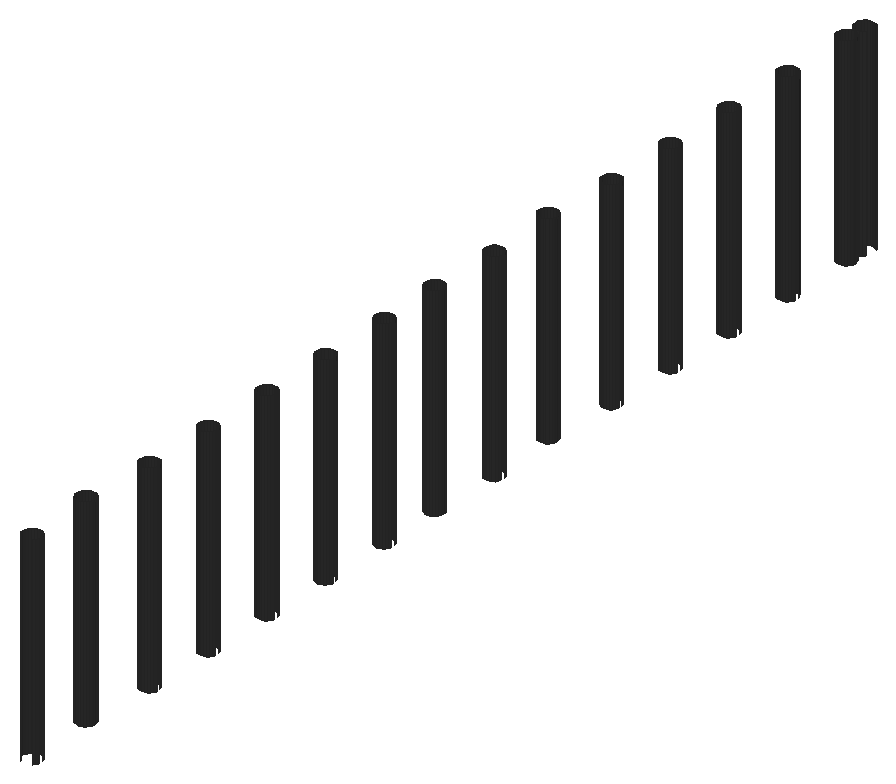
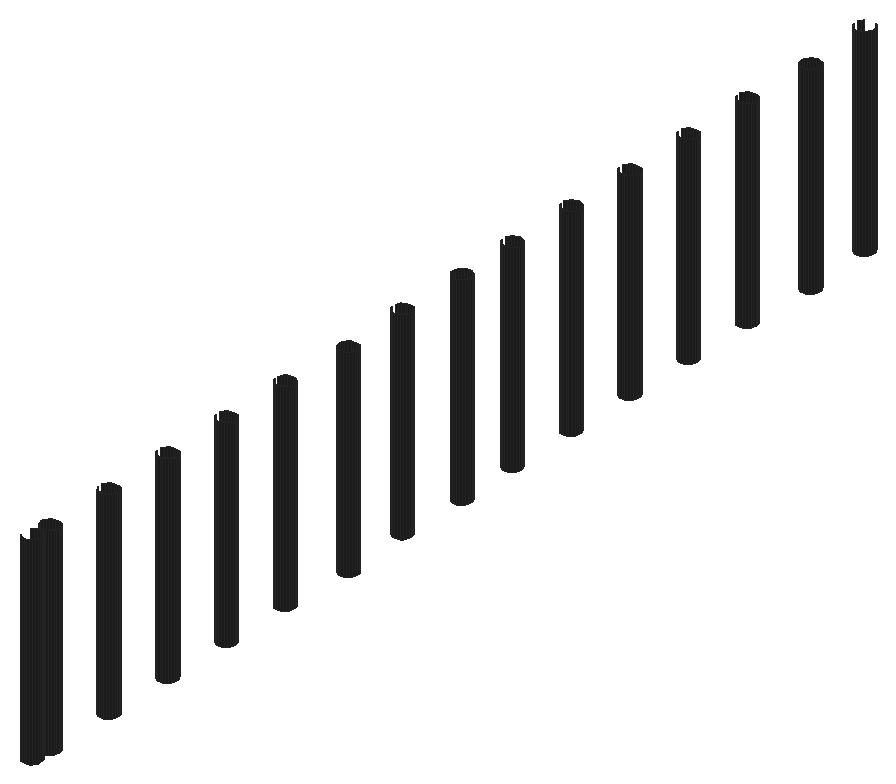
# SketchUp Ruby script. Lengths in inches.
U = 1.inch
M = Sketchup.active_model
def pt(a) = Geom::Point3d.new(a.map { |v| v * U })
def face(e, loops, mat)
  f = e.add_face(loops[0].map { |a| pt(a) })
  loops[1..].each { |l| e.add_face(l.map { |a| pt(a) }).erase! }
  f.material = f.back_material = mat if mat
  f
end
# faces: each face lists its corners as indices into pts; further lists are holes
def faces(e, pts, list, mat = nil) = list.each { |f| face(e, (f[0].is_a?(Array) ? f : [f]).map { |l| l.map { |i| pts[i] } }, mat) }
# xy, xz, yz: faces in a plane at the given z, y or x. An outline is a flat list of corners, or four numbers for a rectangle; further outlines are holes
def ring(l) = l.size == 4 ? [[l[0], l[1]], [l[2], l[1]], [l[2], l[3]], [l[0], l[3]]] : l.each_slice(2).to_a
def flat(e, list, mat, &to3) = list.each { |f| face(e, (f[0].is_a?(Array) ? f : [f]).map { |l| ring(l).map { |u, v| to3.(u, v) } }, mat) }
def xy(e, z, list, mat = nil) = flat(e, list, mat) { |x, y| [x, y, z] }
def xz(e, y, list, mat = nil) = flat(e, list, mat) { |x, z| [x, y, z] }
def yz(e, x, list, mat = nil) = flat(e, list, mat) { |y, z| [x, y, z] }
def lines(e, pts, list) = list.each { |a, b| e.add_line(pt(pts[a]), pt(pts[b])) }
# prism: a flat outline (further loops are holes) pulled along v
def prism(e, loops, v, mat = nil)
  f = face(e, loops, mat); d = Geom::Vector3d.new(v.map { |x| x * U })
  f.pushpull(f.normal.samedirection?(d) ? d.length : -d.length)
end
def box(e, o, s, mat = nil) = prism(e, [[o, [o[0] + s[0], o[1], o[2]], [o[0] + s[0], o[1] + s[1], o[2]], [o[0], o[1] + s[1], o[2]]]], [0, 0, s[2]], mat)
def at(x, y, z, deg = 0) = Geom::Transformation.translation(pt([x, y, z])) * Geom::Transformation.rotation(ORIGIN, Z_AXIS, deg.degrees)
def axes(o, x, y, z) = Geom::Transformation.new([*x, 0, *y, 0, *z, 0, *pt(o).to_a, 1])
def part(name) = M.definitions.add(name)
# library, detail: a bought-in or finely detailed component or shape, given as its bounding box
def library(name, o, s) = part(name).tap { |d| box(d.entities, o, s) }
def detail(e, o, s) = box(e.add_group.entities, o, s)
def put(e, d, t, mat = nil) = e.add_instance(d, t).tap { |i| i.material = mat if mat }
def group(e, t, mat = nil) = e.add_group.tap { |g| g.transformation = t; g.material = mat if mat }.entities
root = M.entities
M.materials.add("[0137_Black]").color = [45, 45, 45]
p = [[2.88,315.04,48],[3.5,314.56,48],[3.5,314.56,113.8],[2.88,315.04,113.8],[2.4,315.66,48],[2.4,315.66,113.8],
  [7.125,315.04,48],[7.6,315.66,48],[7.6,315.66,113.8],[7.125,315.04,113.8],[2.11,316.38,48],[2.11,316.38,113.8],
  [7.9,316.38,48],[7.9,316.38,113.8],[2,317.16,48],[2,317.16,113.8],[2.11,317.93,48],[2.11,317.93,113.8],
  [2.4,318.66,48],[2.4,318.66,113.8],[7.9,317.93,48],[7.6,318.66,48],[7.6,318.66,113.8],[7.9,317.93,113.8],
  [2.88,319.28,48],[2.88,319.28,113.8],[7.125,319.28,48],[7.125,319.28,113.8],[3.5,319.76,48],[3.5,319.76,113.8],
  [6.5,319.76,48],[6.5,319.76,113.8],[4.23,320.06,48],[4.23,320.06,113.8],[4.23,320.06,113.61],[5.78,320.06,48],
  [5.78,320.06,113.8],[5,320.16,48],[5,320.16,113.8],[5,320.16,113.71],[2.67,338.26,48],[3.45,338.16,48],
  [3.45,338.16,113.71],[3.45,338.16,113.8],[2.67,338.26,113.8],[4.23,338.26,48],[4.23,338.26,113.61],[4.23,338.26,113.8],
  [1.95,338.56,48],[1.95,338.56,113.8],[4.95,338.56,48],[4.95,338.56,113.8],[1.33,339.04,48],[1.33,339.04,113.8],
  [5,338.6,48],[5.57,339.04,48],[5.57,339.04,113.8],[0.85,339.66,48],[0.85,339.66,113.8],[6.05,339.66,48],
  [6.05,339.66,113.8],[0.55,340.38,48],[0.55,340.38,113.8],[6.35,340.38,48],[6.35,340.38,113.8],[0.45,341.16,48],
  [0.45,341.16,113.8],[6.45,341.16,48],[6.45,341.16,113.8],[0.55,341.93,48],[0.55,341.93,113.8],[6.35,341.93,48],
  [6.35,341.93,113.8],[0.85,342.66,48],[0.85,342.66,113.8],[6.05,342.66,48],[6.05,342.66,113.8],[1.33,343.28,48],
  [1.33,343.28,113.8],[5.57,343.28,48],[5.57,343.28,113.8],[1.95,343.76,48],[1.95,343.76,113.8],[5,343.72,48],
  [4.95,343.76,48],[4.95,343.76,113.8],[2.67,344.06,48],[2.67,344.06,113.8],[4.23,344.06,48],[4.23,344.06,113.61],
  [4.23,344.06,113.8],[3.45,344.16,48],[3.45,344.16,113.8],[3.45,344.16,113.71],[4.23,362.26,48],[5,362.16,48],
  [5,362.16,113.71],[5,362.16,113.8],[4.23,362.26,113.8],[4.23,362.26,113.61],[5.78,362.26,48],[5.78,362.26,113.8],
  [3.5,362.56,48],[3.5,362.56,113.8],[6.5,362.56,48],[6.5,362.56,113.8],[2.88,363.04,48],[2.88,363.04,113.8],
  [7.125,363.04,48],[7.125,363.04,113.8],[2.4,363.66,48],[2.4,363.66,113.8],[7.6,363.66,48],[7.6,363.66,113.8],
  [2.11,364.38,48],[2.11,364.38,113.8],[7.9,364.38,48],[7.9,364.38,113.8],[2,365.16,48],[2,365.16,113.8],
  [2.11,365.93,48],[2.11,365.93,113.8],[2.4,366.66,48],[2.4,366.66,113.8],[7.9,365.93,48],[7.6,366.66,48],
  [7.6,366.66,113.8],[7.9,365.93,113.8],[2.88,367.28,48],[2.88,367.28,113.8],[7.125,367.28,48],[7.125,367.28,113.8],
  [3.5,367.76,48],[3.5,367.76,113.8],[6.5,367.76,48],[6.5,367.76,113.8],[4.23,368.06,48],[4.23,368.06,113.8],
  [4.23,368.06,113.61],[5.78,368.06,48],[5.78,368.06,113.8],[5,368.16,48],[5,368.16,113.8],[5,368.16,113.71],
  [4.23,386.26,48],[5,386.16,48],[5,386.16,113.71],[5,386.16,113.8],[4.23,386.26,113.8],[4.23,386.26,113.61],
  [5.78,386.26,48],[5.78,386.26,113.8],[3.5,386.56,48],[3.5,386.56,113.8],[6.5,386.56,48],[6.5,386.56,113.8],
  [2.88,387.04,48],[2.88,387.04,113.8],[7.125,387.04,48],[7.125,387.04,113.8],[2.4,387.66,48],[2.4,387.66,113.8],
  [7.6,387.66,48],[7.6,387.66,113.8],[2.11,388.38,48],[2.11,388.38,113.8],[7.9,388.38,48],[7.9,388.38,113.8],
  [2,389.16,48],[2,389.16,113.8],[2.11,389.93,48],[2.11,389.93,113.8],[2.4,390.66,48],[2.4,390.66,113.8],
  [7.9,389.93,48],[7.6,390.66,48],[7.6,390.66,113.8],[7.9,389.93,113.8],[2.88,391.28,48],[2.88,391.28,113.8],
  [7.125,391.28,48],[7.125,391.28,113.8],[3.5,391.76,48],[3.5,391.76,113.8],[6.5,391.76,48],[6.5,391.76,113.8],
  [4.23,392.06,48],[4.23,392.06,113.8],[4.23,392.06,113.61],[5.78,392.06,48],[5.78,392.06,113.8],[5,392.16,48],
  [5,392.16,113.8],[5,392.16,113.71],[4.23,410.26,48],[5,410.16,48],[5,410.16,113.71],[5,410.16,113.8],
  [4.23,410.26,113.8],[4.23,410.26,113.61],[5.78,410.26,48],[5.78,410.26,113.8],[3.5,410.56,48],[3.5,410.56,113.8],
  [6.5,410.56,48],[6.5,410.56,113.8],[2.88,411.04,48],[2.88,411.04,113.8],[7.125,411.04,48],[7.125,411.04,113.8],
  [2.4,411.66,48],[2.4,411.66,113.8],[7.6,411.66,48],[7.6,411.66,113.8],[2.11,412.38,48],[2.11,412.38,113.8],
  [7.9,412.38,48],[7.9,412.38,113.8],[2,413.16,48],[2,413.16,113.8],[2.11,413.93,48],[2.11,413.93,113.8],
  [2.4,414.66,48],[2.4,414.66,113.8],[7.9,413.93,48],[7.6,414.66,48],[7.6,414.66,113.8],[7.9,413.93,113.8],
  [2.88,415.28,48],[2.88,415.28,113.8],[7.125,415.28,48],[7.125,415.28,113.8],[3.5,415.76,48],[3.5,415.76,113.8],
  [6.5,415.76,48],[6.5,415.76,113.8],[4.23,416.06,48],[4.23,416.06,113.8],[4.23,416.06,113.61],[5.78,416.06,48],
  [5.78,416.06,113.8],[5,416.16,48],[5,416.16,113.8],[5,416.16,113.71],[4.23,434.26,48],[5,434.16,48],
  [5,434.16,113.71],[5,434.16,113.8],[4.23,434.26,113.8],[4.23,434.26,113.61],[5.78,434.26,48],[5.78,434.26,113.8],
  [3.5,434.56,48],[3.5,434.56,113.8],[6.5,434.56,48],[6.5,434.56,113.8],[2.88,435.04,48],[2.88,435.04,113.8],
  [7.125,435.04,48],[7.125,435.04,113.8],[2.4,435.66,48],[2.4,435.66,113.8],[7.6,435.66,48],[7.6,435.66,113.8],
  [2.11,436.38,48],[2.11,436.38,113.8],[7.9,436.38,48],[7.9,436.38,113.8],[2,437.16,48],[2,437.16,113.8],
  [2.11,437.93,48],[2.11,437.93,113.8],[2.4,438.66,48],[2.4,438.66,113.8],[7.9,437.93,48],[7.6,438.66,48],
  [7.6,438.66,113.8],[7.9,437.93,113.8],[2.88,439.28,48],[2.88,439.28,113.8],[7.125,439.28,48],[7.125,439.28,113.8],
  [3.5,439.76,48],[3.5,439.76,113.8],[6.5,439.76,48],[6.5,439.76,113.8],[4.23,440.06,48],[4.23,440.06,113.8],
  [4.23,440.06,113.61],[5.78,440.06,48],[5.78,440.06,113.8],[5,440.16,48],[5,440.16,113.8],[5,440.16,113.71],
  [4.23,458.26,48],[5,458.16,48],[5,458.16,113.71],[5,458.16,113.8],[4.23,458.26,113.8],[4.23,458.26,113.61],
  [5.78,458.26,48],[5.78,458.26,113.8],[3.5,458.56,48],[3.5,458.56,113.8],[6.5,458.56,48],[6.5,458.56,113.8],
  [2.88,459.04,48],[2.88,459.04,113.8],[7.125,459.04,48],[7.125,459.04,113.8],[2.4,459.66,48],[2.4,459.66,113.8],
  [7.6,459.66,48],[7.6,459.66,113.8],[2.11,460.38,48],[2.11,460.38,113.8],[7.9,460.38,48],[7.9,460.38,113.8],
  [2,461.16,48],[2,461.16,113.8],[2.11,461.93,48],[2.11,461.93,113.8],[2.4,462.66,48],[2.4,462.66,113.8],
  [7.9,461.93,48],[7.6,462.66,48],[7.6,462.66,113.8],[7.9,461.93,113.8],[2.88,463.28,48],[2.88,463.28,113.8],
  [7.125,463.28,48],[7.125,463.28,113.8],[3.5,463.76,48],[3.5,463.76,113.8],[6.5,463.76,48],[6.5,463.76,113.8],
  [4.23,464.06,48],[4.23,464.06,113.8],[4.23,464.06,113.61],[5.78,464.06,48],[5.78,464.06,113.8],[5,464.16,48],
  [5,464.16,113.8],[5,464.16,113.71],[3.61,479.625,48],[4.38,479.52,48],[4.38,479.52,113.8],[3.61,479.625,113.8],
  [5,479.61,48],[5.16,479.625,48],[5.16,479.625,113.8],[2.88,479.93,48],[2.88,479.93,113.8],[5.88,479.93,48],
  [5.88,479.93,113.8],[2.26,480.4,48],[2.26,480.4,113.8],[6.5,480.4,48],[6.5,480.4,113.8],[1.78,481.02,48],
  [1.78,481.02,113.8],[6.98,481.02,48],[6.98,481.02,113.8],[1.48,481.75,48],[1.48,481.75,113.8],[7.28,481.75,48],
  [7.28,481.75,113.8],[1.38,482.52,48],[1.38,482.52,113.8],[7.38,482.52,48],[7.38,482.52,113.8],[1.48,483.3,48],
  [1.48,483.3,113.8],[7.28,483.3,48],[7.28,483.3,113.8],[1.78,484.02,48],[1.78,484.02,113.8],[6.98,484.02,48],
  [6.98,484.02,113.8],[2.26,484.64,48],[2.26,484.64,113.8],[6.5,484.64,48],[6.5,484.64,113.8],[2.88,485.12,48],
  [2.88,485.12,113.8],[5.88,485.12,48],[5.88,485.12,113.8],[3.61,485.42,48],[3.61,485.42,113.8],[5.16,485.42,48],
  [5.16,485.42,113.8],[4.38,485.52,48],[4.38,485.52,113.8],[5,485.44,48],[4.23,503.15,48],[5,503.05,48],
  [5,503.05,113.71],[5,503.05,113.8],[4.23,503.15,113.8],[4.23,503.15,113.61],[5.78,503.15,48],[5.78,503.15,113.8],
  [3.5,503.45,48],[3.5,503.45,113.8],[6.5,503.45,48],[6.5,503.45,113.8],[2.88,503.93,48],[2.88,503.93,113.8],
  [7.125,503.93,48],[7.125,503.93,113.8],[2.4,504.55,48],[2.4,504.55,113.8],[7.6,504.55,48],[7.6,504.55,113.8],
  [2.11,505.27,48],[2.11,505.27,113.8],[7.9,505.27,48],[7.9,505.27,113.8],[2,506.05,48],[2,506.05,113.8],
  [2.11,506.82,48],[2.11,506.82,113.8],[2.4,507.55,48],[2.4,507.55,113.8],[7.9,506.82,48],[7.6,507.55,48],
  [7.6,507.55,113.8],[7.9,506.82,113.8],[2.88,508.17,48],[2.88,508.17,113.8],[7.125,508.17,48],[7.125,508.17,113.8],
  [3.5,508.64,48],[3.5,508.64,113.8],[6.5,508.64,48],[6.5,508.64,113.8],[4.23,508.94,48],[4.23,508.94,113.8],
  [4.23,508.94,113.61],[5.78,508.94,48],[5.78,508.94,113.8],[5,509.05,48],[5,509.05,113.8],[5,509.05,113.71],
  [2.67,527.15,48],[3.45,527.05,48],[3.45,527.05,113.71],[3.45,527.05,113.8],[2.67,527.15,113.8],[4.23,527.15,48],
  [4.23,527.15,113.61],[4.23,527.15,113.8],[1.95,527.45,48],[1.95,527.45,113.8],[4.95,527.45,48],[4.95,527.45,113.8],
  [1.33,527.93,48],[1.33,527.93,113.8],[5,527.49,48],[5.57,527.93,48],[5.57,527.93,113.8],[0.85,528.55,48],
  [0.85,528.55,113.8],[6.05,528.55,48],[6.05,528.55,113.8],[0.55,529.27,48],[0.55,529.27,113.8],[6.35,529.27,48],
  [6.35,529.27,113.8],[0.45,530.05,48],[0.45,530.05,113.8],[6.45,530.05,48],[6.45,530.05,113.8],[0.55,530.82,48],
  [0.55,530.82,113.8],[6.35,530.82,48],[6.35,530.82,113.8],[0.85,531.55,48],[0.85,531.55,113.8],[6.05,531.55,48],
  [6.05,531.55,113.8],[1.33,532.17,48],[1.33,532.17,113.8],[5.57,532.17,48],[5.57,532.17,113.8],[1.95,532.64,48],
  [1.95,532.64,113.8],[5,532.6,48],[4.95,532.64,48],[4.95,532.64,113.8],[2.67,532.94,48],[2.67,532.94,113.8],
  [4.23,532.94,48],[4.23,532.94,113.61],[4.23,532.94,113.8],[3.45,533.05,48],[3.45,533.05,113.8],[3.45,533.05,113.71],
  [4.23,551.15,48],[5,551.05,48],[5,551.05,113.71],[5,551.05,113.8],[4.23,551.15,113.8],[4.23,551.15,113.61],
  [5.78,551.15,48],[5.78,551.15,113.8],[3.5,551.45,48],[3.5,551.45,113.8],[6.5,551.45,48],[6.5,551.45,113.8],
  [2.88,551.93,48],[2.88,551.93,113.8],[7.125,551.93,48],[7.125,551.93,113.8],[2.4,552.55,48],[2.4,552.55,113.8],
  [7.6,552.55,48],[7.6,552.55,113.8],[2.11,553.27,48],[2.11,553.27,113.8],[7.9,553.27,48],[7.9,553.27,113.8],
  [2,554.05,48],[2,554.05,113.8],[2.11,554.82,48],[2.11,554.82,113.8],[2.4,555.55,48],[2.4,555.55,113.8],
  [7.9,554.82,48],[7.6,555.55,48],[7.6,555.55,113.8],[7.9,554.82,113.8],[2.88,556.17,48],[2.88,556.17,113.8],
  [7.125,556.17,48],[7.125,556.17,113.8],[3.5,556.64,48],[3.5,556.64,113.8],[6.5,556.64,48],[6.5,556.64,113.8],
  [4.23,556.94,48],[4.23,556.94,113.8],[4.23,556.94,113.61],[5.78,556.94,48],[5.78,556.94,113.8],[5,557.05,48],
  [5,557.05,113.8],[5,557.05,113.71],[4.23,575.15,48],[5,575.05,48],[5,575.05,113.71],[5,575.05,113.8],
  [4.23,575.15,113.8],[4.23,575.15,113.61],[5.78,575.15,48],[5.78,575.15,113.8],[3.5,575.45,48],[3.5,575.45,113.8],
  [6.5,575.45,48],[6.5,575.45,113.8],[2.88,575.93,48],[2.88,575.93,113.8],[7.125,575.93,48],[7.125,575.93,113.8],
  [2.4,576.55,48],[2.4,576.55,113.8],[7.6,576.55,48],[7.6,576.55,113.8],[2.11,577.27,48],[2.11,577.27,113.8],
  [7.9,577.27,48],[7.9,577.27,113.8],[2,578.05,48],[2,578.05,113.8],[2.11,578.82,48],[2.11,578.82,113.8],
  [2.4,579.55,48],[2.4,579.55,113.8],[7.9,578.82,48],[7.6,579.55,48],[7.6,579.55,113.8],[7.9,578.82,113.8],
  [2.88,580.17,48],[2.88,580.17,113.8],[7.125,580.17,48],[7.125,580.17,113.8],[3.5,580.64,48],[3.5,580.64,113.8],
  [6.5,580.64,48],[6.5,580.64,113.8],[4.23,580.94,48],[4.23,580.94,113.8],[4.23,580.94,113.61],[5.78,580.94,48],
  [5.78,580.94,113.8],[5,581.05,48],[5,581.05,113.8],[5,581.05,113.71],[4.23,599.15,48],[5,599.05,48],
  [5,599.05,113.71],[5,599.05,113.8],[4.23,599.15,113.8],[4.23,599.15,113.61],[5.78,599.15,48],[5.78,599.15,113.8],
  [3.5,599.45,48],[3.5,599.45,113.8],[6.5,599.45,48],[6.5,599.45,113.8],[2.88,599.93,48],[2.88,599.93,113.8],
  [7.125,599.93,48],[7.125,599.93,113.8],[2.4,600.55,48],[2.4,600.55,113.8],[7.6,600.55,48],[7.6,600.55,113.8],
  [2.11,601.27,48],[2.11,601.27,113.8],[7.9,601.27,48],[7.9,601.27,113.8],[2,602.05,48],[2,602.05,113.8],
  [2.11,602.82,48],[2.11,602.82,113.8],[2.4,603.55,48],[2.4,603.55,113.8],[7.9,602.82,48],[7.6,603.55,48],
  [7.6,603.55,113.8],[7.9,602.82,113.8],[2.88,604.17,48],[2.88,604.17,113.8],[7.125,604.17,48],[7.125,604.17,113.8],
  [3.5,604.64,48],[3.5,604.64,113.8],[6.5,604.64,48],[6.5,604.64,113.8],[4.23,604.94,48],[4.23,604.94,113.8],
  [4.23,604.94,113.61],[5.78,604.94,48],[5.78,604.94,113.8],[5,605.05,48],[5,605.05,113.8],[5,605.05,113.71],
  [4.23,623.15,48],[5,623.05,48],[5,623.05,113.71],[5,623.05,113.8],[4.23,623.15,113.8],[4.23,623.15,113.61],
  [5.78,623.15,48],[5.78,623.15,113.8],[3.5,623.45,48],[3.5,623.45,113.8],[6.5,623.45,48],[6.5,623.45,113.8],
  [2.88,623.93,48],[2.88,623.93,113.8],[7.125,623.93,48],[7.125,623.93,113.8],[2.4,624.55,48],[2.4,624.55,113.8],
  [7.6,624.55,48],[7.6,624.55,113.8],[2.11,625.27,48],[2.11,625.27,113.8],[7.9,625.27,48],[7.9,625.27,113.8],
  [2,626.05,48],[2,626.05,113.8],[2.11,626.82,48],[2.11,626.82,113.8],[2.4,627.55,48],[2.4,627.55,113.8],
  [7.9,626.82,48],[7.6,627.55,48],[7.6,627.55,113.8],[7.9,626.82,113.8],[2.88,628.17,48],[2.88,628.17,113.8],
  [7.125,628.17,48],[7.125,628.17,113.8],[3.5,628.64,48],[3.5,628.64,113.8],[6.5,628.64,48],[6.5,628.64,113.8],
  [4.23,628.94,48],[4.23,628.94,113.8],[4.23,628.94,113.61],[5.78,628.94,48],[5.78,628.94,113.8],[5,629.05,48],
  [5,629.05,113.8],[5,629.05,113.71],[4.23,647.15,48],[5,647.05,48],[5,647.05,113.71],[5,647.05,113.8],
  [4.23,647.15,113.8],[4.23,647.15,113.61],[5.78,647.15,48],[5.78,647.15,113.8],[3.5,647.45,48],[3.5,647.45,113.8],
  [6.5,647.45,48],[6.5,647.45,113.8],[2.88,647.93,48],[2.88,647.93,113.8],[7.125,647.93,48],[7.125,647.93,113.8],
  [2.4,648.55,48],[2.4,648.55,113.8],[7.6,648.55,48],[7.6,648.55,113.8],[2.11,649.27,48],[2.11,649.27,113.8],
  [7.9,649.27,48],[7.9,649.27,113.8],[2,650.05,48],[2,650.05,113.8],[8,650.05,48],[8,650.05,113.8],
  [2.11,650.82,48],[2.11,650.82,113.8],[2.4,651.55,48],[2.4,651.55,113.8],[7.9,650.82,48],[7.6,651.55,48],
  [7.6,651.55,113.8],[7.9,650.82,113.8],[2.88,652.17,48],[2.88,652.17,113.8],[7.125,652.17,48],[7.125,652.17,113.8],
  [3.5,652.64,48],[3.5,652.64,113.8],[6.5,652.64,48],[6.5,652.64,113.8],[4.23,652.94,48],[4.23,652.94,113.8],
  [4.23,652.94,113.61],[5.78,652.94,48],[5.78,652.94,113.8],[5,653.05,48],[5,653.05,113.8],[4.86,653.82,48],
  [5.63,653.72,48],[5.63,653.72,113.8],[4.86,653.82,113.8],[6.41,653.82,48],[6.41,653.82,113.8],[4.13,654.12,48],
  [4.13,654.12,113.8],[7.13,654.12,48],[7.13,654.12,113.8],[3.51,654.6,48],[3.51,654.6,113.8],[7.76,654.6,48],
  [7.76,654.6,113.8],[3.04,655.22,48],[3.04,655.22,113.8],[2.74,655.94,48],[2.74,655.94,113.8],[2.74,655.94,113.61],
  [2.63,656.72,48],[2.63,656.72,113.8],[2.74,657.5,48],[2.74,657.5,113.8],[3.04,658.22,48],[3.04,658.22,113.8],
  [3.51,658.84,48],[3.51,658.84,113.8],[4.13,659.32,48],[4.13,659.32,113.8],[7.76,658.84,48],[7.13,659.32,48],
  [7.13,659.32,113.8],[7.76,658.84,113.8],[4.86,659.62,48],[4.86,659.62,113.8],[6.41,659.62,48],[6.41,659.62,113.8],
  [5.63,659.72,48],[5.63,659.72,113.8]]
faces(root,p,[[0,1,2,3],[4,0,3,5],[6,7,8,9],[10,4,5,11],[7,12,13,8],[14,10,11,15],[16,14,15,17],[18,16,17,19],
  [20,21,22,23],[24,18,19,25],[21,26,27,22],[28,24,25,29],[26,30,31,27],[32,28,29,33,34],[30,35,36,31],[37,32,34,33,38,39],
  [35,37,39,38,36],[40,41,42,43,44],[41,45,46,47,43,42],[48,40,44,49],[45,50,51,47,46],[52,48,49,53],[50,54,55,56,51],[57,52,53,58],
  [55,59,60,56],[61,57,58,62],[59,63,64,60],[65,61,62,66],[63,67,68,64],[69,65,66,70],[67,71,72,68],[73,69,70,74],
  [71,75,76,72],[77,73,74,78],[75,79,80,76],[81,77,78,82],[79,83,84,85,80],[86,81,82,87],[84,88,89,90,85],[91,86,87,92,93],
  [88,91,93,92,90,89],[94,95,96,97,98,99],[95,100,101,97,96],[102,94,99,98,103],[100,104,105,101],[106,102,103,107],[104,108,109,105],[110,106,107,111],
  [108,112,113,109],[114,110,111,115],[112,116,117,113],[118,114,115,119],[120,118,119,121],[122,120,121,123],[124,125,126,127],[128,122,123,129],
  [125,130,131,126],[132,128,129,133],[130,134,135,131],[136,132,133,137,138],[134,139,140,135],[141,136,138,137,142,143],[139,141,143,142,140],[144,145,146,147,148,149],
  [145,150,151,147,146],[152,144,149,148,153],[150,154,155,151],[156,152,153,157],[154,158,159,155],[160,156,157,161],[158,162,163,159],[164,160,161,165],
  [162,166,167,163],[168,164,165,169],[170,168,169,171],[172,170,171,173],[174,175,176,177],[178,172,173,179],[175,180,181,176],[182,178,179,183],
  [180,184,185,181],[186,182,183,187,188],[184,189,190,185],[191,186,188,187,192,193],[189,191,193,192,190],[194,195,196,197,198,199],[195,200,201,197,196],[202,194,199,198,203],
  [200,204,205,201],[206,202,203,207],[204,208,209,205],[210,206,207,211],[208,212,213,209],[214,210,211,215],[212,216,217,213],[218,214,215,219],
  [220,218,219,221],[222,220,221,223],[224,225,226,227],[228,222,223,229],[225,230,231,226],[232,228,229,233],[230,234,235,231],[236,232,233,237,238],
  [234,239,240,235],[241,236,238,237,242,243],[239,241,243,242,240],[244,245,246,247,248,249],[245,250,251,247,246],[252,244,249,248,253],[250,254,255,251],[256,252,253,257],
  [254,258,259,255],[260,256,257,261],[258,262,263,259],[264,260,261,265],[262,266,267,263],[268,264,265,269],[270,268,269,271],[272,270,271,273],
  [274,275,276,277],[278,272,273,279],[275,280,281,276],[282,278,279,283],[280,284,285,281],[286,282,283,287,288],[284,289,290,285],[291,286,288,287,292,293],
  [289,291,293,292,290],[294,295,296,297,298,299],[295,300,301,297,296],[302,294,299,298,303],[300,304,305,301],[306,302,303,307],[304,308,309,305],[310,306,307,311],
  [308,312,313,309],[314,310,311,315],[312,316,317,313],[318,314,315,319],[320,318,319,321],[322,320,321,323],[324,325,326,327],[328,322,323,329],
  [325,330,331,326],[332,328,329,333],[330,334,335,331],[336,332,333,337,338],[334,339,340,335],[341,336,338,337,342,343],[339,341,343,342,340],[344,345,346,347],
  [345,348,349,350,346],[351,344,347,352],[349,353,354,350],[355,351,352,356],[353,357,358,354],[359,355,356,360],[357,361,362,358],[363,359,360,364],
  [361,365,366,362],[367,363,364,368],[365,369,370,366],[371,367,368,372],[369,373,374,370],[375,371,372,376],[373,377,378,374],[379,375,376,380],
  [377,381,382,378],[383,379,380,384],[381,385,386,382],[387,383,384,388],[385,389,390,386],[391,387,388,392],[389,393,391,392,390],[394,395,396,397,398,399],
  [395,400,401,397,396],[402,394,399,398,403],[400,404,405,401],[406,402,403,407],[404,408,409,405],[410,406,407,411],[408,412,413,409],[414,410,411,415],
  [412,416,417,413],[418,414,415,419],[420,418,419,421],[422,420,421,423],[424,425,426,427],[428,422,423,429],[425,430,431,426],[432,428,429,433],
  [430,434,435,431],[436,432,433,437,438],[434,439,440,435],[441,436,438,437,442,443],[439,441,443,442,440],[444,445,446,447,448],[445,449,450,451,447,446],[452,444,448,453],
  [449,454,455,451,450],[456,452,453,457],[454,458,459,460,455],[461,456,457,462],[459,463,464,460],[465,461,462,466],[463,467,468,464],[469,465,466,470],
  [467,471,472,468],[473,469,470,474],[471,475,476,472],[477,473,474,478],[475,479,480,476],[481,477,478,482],[479,483,484,480],[485,481,482,486],
  [483,487,488,489,484],[490,485,486,491],[488,492,493,494,489],[495,490,491,496,497],[492,495,497,496,494,493],[498,499,500,501,502,503],[499,504,505,501,500],[506,498,503,502,507],
  [504,508,509,505],[510,506,507,511],[508,512,513,509],[514,510,511,515],[512,516,517,513],[518,514,515,519],[516,520,521,517],[522,518,519,523],
  [524,522,523,525],[526,524,525,527],[528,529,530,531],[532,526,527,533],[529,534,535,530],[536,532,533,537],[534,538,539,535],[540,536,537,541,542],
  [538,543,544,539],[545,540,542,541,546,547],[543,545,547,546,544],[548,549,550,551,552,553],[549,554,555,551,550],[556,548,553,552,557],[554,558,559,555],[560,556,557,561],
  [558,562,563,559],[564,560,561,565],[562,566,567,563],[568,564,565,569],[566,570,571,567],[572,568,569,573],[574,572,573,575],[576,574,575,577],
  [578,579,580,581],[582,576,577,583],[579,584,585,580],[586,582,583,587],[584,588,589,585],[590,586,587,591,592],[588,593,594,589],[595,590,592,591,596,597],
  [593,595,597,596,594],[598,599,600,601,602,603],[599,604,605,601,600],[606,598,603,602,607],[604,608,609,605],[610,606,607,611],[608,612,613,609],[614,610,611,615],
  [612,616,617,613],[618,614,615,619],[616,620,621,617],[622,618,619,623],[624,622,623,625],[626,624,625,627],[628,629,630,631],[632,626,627,633],
  [629,634,635,630],[636,632,633,637],[634,638,639,635],[640,636,637,641,642],[638,643,644,639],[645,640,642,641,646,647],[643,645,647,646,644],[648,649,650,651,652,653],
  [649,654,655,651,650],[656,648,653,652,657],[654,658,659,655],[660,656,657,661],[658,662,663,659],[664,660,661,665],[662,666,667,663],[668,664,665,669],
  [666,670,671,667],[672,668,669,673],[674,672,673,675],[676,674,675,677],[678,679,680,681],[682,676,677,683],[679,684,685,680],[686,682,683,687],
  [684,688,689,685],[690,686,687,691,692],[688,693,694,689],[695,690,692,691,696,697],[693,695,697,696,694],[698,699,700,701,702,703],[699,704,705,701,700],[706,698,703,702,707],
  [704,708,709,705],[710,706,707,711],[708,712,713,709],[714,710,711,715],[712,716,717,713],[718,714,715,719],[716,720,721,717],[722,718,719,723],
  [720,724,725,721],[726,722,723,727],[728,726,727,729],[730,731,732,733],[734,728,729,735],[731,736,737,732],[738,734,735,739],[736,740,741,737],
  [742,738,739,743,744],[740,745,746,741],[747,742,744,743,748],[745,747,748,746],[749,750,751,752],[750,753,754,751],[755,749,752,756],[753,757,758,754],
  [759,755,756,760],[757,761,762,758],[763,759,760,764],[765,763,764,766,767],[768,765,767,766,769],[770,768,769,771],[772,770,771,773],[774,772,773,775],
  [776,774,775,777],[778,779,780,781],[782,776,777,783],[779,784,785,780],[786,782,783,787],[784,786,787,785]],"[0137_Black]")
